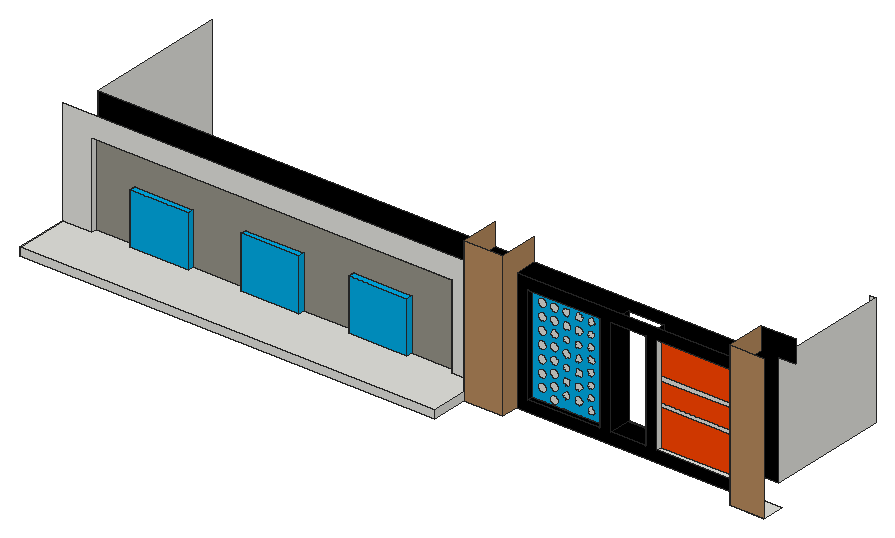
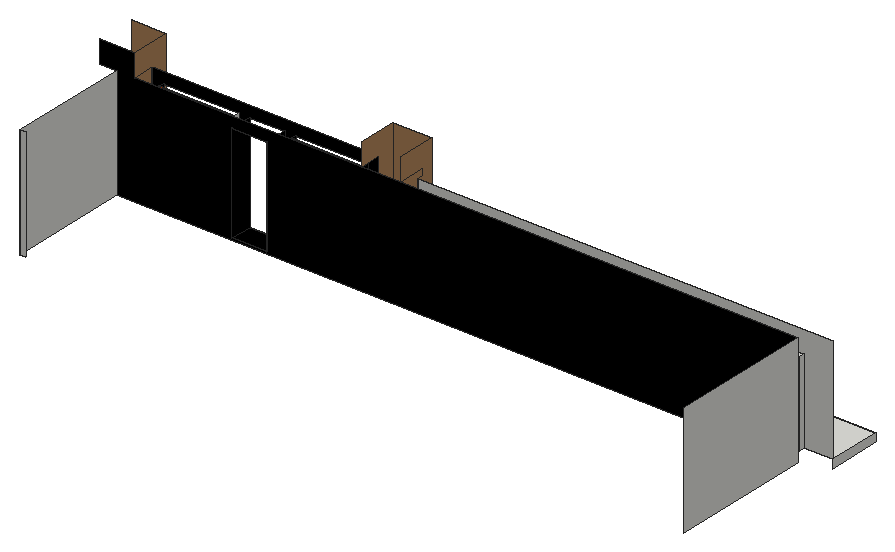
# SketchUp Ruby script. Lengths in inches.
U = 1.inch
M = Sketchup.active_model
def pt(a) = Geom::Point3d.new(a.map { |v| v * U })
def face(e, loops, mat)
  f = e.add_face(loops[0].map { |a| pt(a) })
  loops[1..].each { |l| e.add_face(l.map { |a| pt(a) }).erase! }
  f.material = f.back_material = mat if mat
  f
end
# faces: each face lists its corners as indices into pts; further lists are holes
def faces(e, pts, list, mat = nil) = list.each { |f| face(e, (f[0].is_a?(Array) ? f : [f]).map { |l| l.map { |i| pts[i] } }, mat) }
# xy, xz, yz: faces in a plane at the given z, y or x. An outline is a flat list of corners, or four numbers for a rectangle; further outlines are holes
def ring(l) = l.size == 4 ? [[l[0], l[1]], [l[2], l[1]], [l[2], l[3]], [l[0], l[3]]] : l.each_slice(2).to_a
def flat(e, list, mat, &to3) = list.each { |f| face(e, (f[0].is_a?(Array) ? f : [f]).map { |l| ring(l).map { |u, v| to3.(u, v) } }, mat) }
def xy(e, z, list, mat = nil) = flat(e, list, mat) { |x, y| [x, y, z] }
def xz(e, y, list, mat = nil) = flat(e, list, mat) { |x, z| [x, y, z] }
def yz(e, x, list, mat = nil) = flat(e, list, mat) { |y, z| [x, y, z] }
def lines(e, pts, list) = list.each { |a, b| e.add_line(pt(pts[a]), pt(pts[b])) }
# prism: a flat outline (further loops are holes) pulled along v
def prism(e, loops, v, mat = nil)
  f = face(e, loops, mat); d = Geom::Vector3d.new(v.map { |x| x * U })
  f.pushpull(f.normal.samedirection?(d) ? d.length : -d.length)
end
def box(e, o, s, mat = nil) = prism(e, [[o, [o[0] + s[0], o[1], o[2]], [o[0] + s[0], o[1] + s[1], o[2]], [o[0], o[1] + s[1], o[2]]]], [0, 0, s[2]], mat)
def at(x, y, z, deg = 0) = Geom::Transformation.translation(pt([x, y, z])) * Geom::Transformation.rotation(ORIGIN, Z_AXIS, deg.degrees)
def axes(o, x, y, z) = Geom::Transformation.new([*x, 0, *y, 0, *z, 0, *pt(o).to_a, 1])
def part(name) = M.definitions.add(name)
# library, detail: a bought-in or finely detailed component or shape, given as its bounding box
def library(name, o, s) = part(name).tap { |d| box(d.entities, o, s) }
def detail(e, o, s) = box(e.add_group.entities, o, s)
def put(e, d, t, mat = nil) = e.add_instance(d, t).tap { |i| i.material = mat if mat }
def group(e, t, mat = nil) = e.add_group.tap { |g| g.transformation = t; g.material = mat if mat }.entities
root = M.entities
M.materials.add("Niraj_Shoe_Stitching").color = [181, 137, 92]
M.materials.add("[0024_OrangeRed]").color = [255, 69, 0]
M.materials.add("[0097_DeepSkyBlue]1").color = [0, 171, 229]
M.materials.add("[0137_Black]").color = [0, 0, 0]
M.materials.add("[Formica Graystone]").color = [149, 146, 135]
xy(root,-4.9375,[[365.58,19.875,384,31.875]])
xy(root,-0.56,[[0,0,222.65,0,222.65,28.875,208.96,28.875,208.96,31.875,185.04,31.875,185.04,28.875,153.73,28.875,153.73,31.875,126.98,31.875,126.98,28.875,95.67,28.875,95.67,31.875,67.42,31.875,67.42,28.875,36.1,28.875,36.1,31.875,15.47,31.875,15.47,28.875,0,28.875]])
xy(root,1.0625,[[319.08,28.875,359.58,31.875]])
xy(root,1.0625,[[249.65,28.875,288.24,31.875],[294.24,28.875,313.08,40.875]],"[0137_Black]")
xy(root,27.07,[[36.1,28.875,67.42,31.875],[95.67,28.875,126.98,31.875],[153.73,28.875,185.04,31.875]],"[0097_DeepSkyBlue]1")
xy(root,44.57,[[15.47,28.875,208.96,31.875]])
xz(root,0,[[0,-4.9375,222.65,-0.56]])
xz(root,19.875,[[222.65,-4.9375,243.65,72],[365.58,-4.9375,384,72]],"Niraj_Shoe_Stitching")
xz(root,28.875,[[0,-0.56,15.47,-0.56,15.47,44.57,208.96,44.57,208.96,-0.56,222.65,-0.56,222.65,56.2,0,56.2]])
xz(root,28.875,[[36.1,-0.56,67.42,27.07],[95.67,-0.56,126.98,27.07],[153.73,-0.56,185.04,27.07]],"[0097_DeepSkyBlue]1")
xz(root,28.875,[[[243.65,-4.9375,365.58,60],[319.08,1.0625,359.58,54],[249.65,1.0625,288.24,54],[294.24,1.0625,313.08,54]]],"[0137_Black]")
xz(root,31.875,[[281.13,-2.54,281.62,-2.54,282.09,-2.42,282.52,-2.18,282.87,-1.83,283.11,-1.41,283.24,-0.9375,283.24,-0.45,283.12,0.03,282.875,0.45,282.53,0.8,282.11,1.05,282.05,1.0625,280.71,1.0625,280.67,1.05,280.25,0.81,279.9,0.46,279.65,0.04,279.53,-0.43,279.52,-0.92,279.65,-1.39,279.89,-1.82,280.24,-2.17,280.66,-2.41],[254.88,-1.23,255.37,-1.23,255.84,-1.11,256.27,-0.86,256.62,-0.52,256.86,-0.1,256.99,0.375,256.99,0.87,256.94,1.0625,253.33,1.0625,253.28,0.88,253.27,0.39,253.4,-0.08,253.64,-0.51,253.99,-0.85,254.41,-1.1],[274.57,-0.79,275.06,-0.79,275.53,-0.67,275.96,-0.43,276.3,-0.08,276.55,0.34,276.68,0.8125,276.68,1.0625,272.96,1.0625,272.96,0.83,273.09,0.36,273.33,-0.07,273.67,-0.42,274.1,-0.66],[268.5,-0.36,268.97,-0.23,269.39,0.01,269.74,0.36,269.99,0.78,270.07,1.0625,266.45,1.0625,266.52,0.79,266.77,0.37,267.11,0.02,267.53,-0.22,268.01,-0.35],[261.44,1.83,261.93,1.83,262.41,1.96,262.83,2.2,263.18,2.54,263.43,2.97,263.55,3.4375,263.56,3.93,263.43,4.4,263.1875,4.83,262.84,5.17,262.42,5.42,261.95,5.55,261.46,5.55,260.99,5.43,260.5625,5.18,260.21,4.84,259.97,4.42,259.84,3.94,259.84,3.46,259.96,2.98,260.2,2.56,260.55,2.21,260.97,1.96],
  [281.13,3.58,281.62,3.58,282.09,3.71,282.52,3.95,282.87,4.29,283.11,4.72,283.24,5.1875,283.24,5.68,283.12,6.15,282.875,6.58,282.53,6.92,282.11,7.17,281.64,7.3,281.15,7.3,280.67,7.18,280.25,6.93,279.9,6.59,279.65,6.17,279.53,5.69,279.52,5.21,279.65,4.73,279.89,4.31,280.24,3.96,280.66,3.71],[254.88,5.58,255.37,5.58,255.84,5.71,256.27,5.95,256.62,6.29,256.86,6.72,256.99,7.1875,256.99,7.68,256.87,8.15,256.625,8.58,256.28,8.92,255.86,9.17,255.39,9.3,254.9,9.3,254.42,9.18,254,8.93,253.65,8.59,253.4,8.17,253.28,7.69,253.27,7.21,253.4,6.73,253.64,6.31,253.99,5.96,254.41,5.71],[274.57,5.96,275.06,5.96,275.53,6.08,275.96,6.32,276.3,6.67,276.55,7.09,276.68,7.5625,276.68,8.05,276.56,8.53,276.3125,8.95,275.97,9.3,275.55,9.55,275.07,9.68,274.58,9.68,274.11,9.55,273.6875,9.31,273.34,8.96,273.09,8.54,272.96,8.07,272.96,7.58,273.09,7.11,273.33,6.68,273.67,6.33,274.1,6.09],[268.01,6.33,268.5,6.33,268.97,6.46,269.39,6.7,269.74,7.04,269.99,7.47,270.12,7.9375,270.12,8.43,269.99,8.9,269.75,9.33,269.41,9.67,268.98,9.92,268.51,10.05,268.02,10.05,267.55,9.93,267.125,9.68,266.78,9.34,266.53,8.92,266.4,8.44,266.4,7.96,266.52,7.48,266.77,7.06,267.11,6.71,267.53,6.46],[261.44,8.21,261.93,8.21,262.41,8.33,262.83,8.57,263.18,8.92,263.43,9.34,263.55,9.8125,263.56,10.3,263.43,10.78,263.1875,11.2,262.84,11.55,262.42,11.8,261.95,11.93,261.46,11.93,260.99,11.8,260.5625,11.56,260.21,11.21,259.97,10.79,259.84,10.32,259.84,9.83,259.96,9.36,260.2,8.93,260.55,8.58,260.97,8.34],
  [281.13,9.71,281.62,9.71,282.09,9.83,282.52,10.07,282.87,10.42,283.11,10.84,283.24,11.3125,283.24,11.8,283.12,12.28,282.875,12.7,282.53,13.05,282.11,13.3,281.64,13.43,281.15,13.43,280.67,13.3,280.25,13.06,279.9,12.71,279.65,12.29,279.53,11.82,279.52,11.33,279.65,10.86,279.89,10.43,280.24,10.08,280.66,9.84],[255.37,12.39,255.84,12.52,256.27,12.76,256.62,13.11,256.86,13.53,256.99,14,256.99,14.49,256.87,14.96,256.625,15.39,256.28,15.74,255.86,15.98,255.39,16.11,254.9,16.11,254.42,15.99,254,15.75,253.65,15.4,253.4,14.98,253.28,14.51,253.27,14.02,253.4,13.54,253.64,13.12,253.99,12.77,254.41,12.53,254.88,12.4],[274.57,12.71,275.06,12.71,275.53,12.83,275.96,13.07,276.3,13.42,276.55,13.84,276.68,14.3125,276.68,14.8,276.56,15.28,276.3125,15.7,275.97,16.05,275.55,16.3,275.07,16.43,274.58,16.43,274.11,16.3,273.6875,16.06,273.34,15.71,273.09,15.29,272.96,14.82,272.96,14.33,273.09,13.86,273.33,13.43,273.67,13.08,274.1,12.84],[268.01,13.02,268.5,13.02,268.97,13.14,269.39,13.39,269.74,13.73,269.99,14.15,270.12,14.625,270.12,15.12,269.99,15.59,269.75,16.01,269.41,16.36,268.98,16.61,268.51,16.74,268.02,16.74,267.55,16.61,267.125,16.37,266.78,16.03,266.53,15.6,266.4,15.13,266.4,14.64,266.52,14.17,266.77,13.74,267.11,13.4,267.53,13.15],[261.44,14.58,261.93,14.58,262.41,14.71,262.83,14.95,263.18,15.29,263.43,15.72,263.55,16.1875,263.56,16.68,263.43,17.15,263.1875,17.58,262.84,17.92,262.42,18.17,261.95,18.3,261.46,18.3,260.99,18.18,260.5625,17.93,260.21,17.59,259.97,17.17,259.84,16.69,259.84,16.21,259.96,15.73,260.2,15.31,260.55,14.96,260.97,14.71],
  [281.13,15.83,281.62,15.83,282.09,15.96,282.52,16.2,282.87,16.54,283.11,16.97,283.24,17.4375,283.24,17.93,283.12,18.4,282.875,18.83,282.53,19.17,282.11,19.42,281.64,19.55,281.15,19.55,280.67,19.43,280.25,19.18,279.9,18.84,279.65,18.42,279.53,17.94,279.52,17.46,279.65,16.98,279.89,16.56,280.24,16.21,280.66,15.96],[254.88,19.21,255.37,19.21,255.84,19.33,256.27,19.57,256.62,19.92,256.86,20.34,256.99,20.8125,256.99,21.3,256.87,21.78,256.625,22.2,256.28,22.55,255.86,22.8,255.39,22.93,254.9,22.93,254.42,22.8,254,22.56,253.65,22.21,253.4,21.79,253.28,21.32,253.27,20.83,253.4,20.36,253.64,19.93,253.99,19.58,254.41,19.34],[274.57,19.46,275.06,19.46,275.53,19.58,275.96,19.82,276.3,20.17,276.55,20.59,276.68,21.0625,276.68,21.55,276.56,22.03,276.3125,22.45,275.97,22.8,275.55,23.05,275.07,23.18,274.58,23.18,274.11,23.05,273.6875,22.81,273.34,22.46,273.09,22.04,272.96,21.57,272.96,21.08,273.09,20.61,273.33,20.18,273.67,19.83,274.1,19.59],[268.01,19.71,268.5,19.71,268.97,19.83,269.39,20.07,269.74,20.42,269.99,20.84,270.12,21.3125,270.12,21.8,269.99,22.28,269.75,22.7,269.41,23.05,268.98,23.3,268.51,23.43,268.02,23.43,267.55,23.3,267.125,23.06,266.78,22.71,266.53,22.29,266.4,21.82,266.4,21.33,266.52,20.86,266.77,20.43,267.11,20.08,267.53,19.84],[319.08,20.45,359.58,22.56],
  [261.44,20.96,261.93,20.96,262.41,21.08,262.83,21.32,263.18,21.67,263.43,22.09,263.55,22.5625,263.56,23.05,263.43,23.53,263.1875,23.95,262.84,24.3,262.42,24.55,261.95,24.68,261.46,24.68,260.99,24.55,260.5625,24.31,260.21,23.96,259.97,23.54,259.84,23.07,259.84,22.58,259.96,22.11,260.2,21.68,260.55,21.33,260.97,21.09],[281.13,21.96,281.62,21.96,282.09,22.08,282.52,22.32,282.87,22.67,283.11,23.09,283.24,23.5625,283.24,24.05,283.12,24.53,282.875,24.95,282.53,25.3,282.11,25.55,281.64,25.68,281.15,25.68,280.67,25.55,280.25,25.31,279.9,24.96,279.65,24.54,279.53,24.07,279.52,23.58,279.65,23.11,279.89,22.68,280.24,22.33,280.66,22.09],[254.88,26.02,255.37,26.02,255.84,26.14,256.27,26.39,256.62,26.73,256.86,27.15,256.99,27.625,256.99,28.12,256.87,28.59,256.625,29.01,256.28,29.36,255.86,29.61,255.39,29.74,254.9,29.74,254.42,29.61,254,29.37,253.65,29.03,253.4,28.6,253.28,28.13,253.27,27.64,253.4,27.17,253.64,26.74,253.99,26.4,254.41,26.15],[274.57,26.21,275.06,26.21,275.53,26.33,275.96,26.57,276.3,26.92,276.55,27.34,276.68,27.8125,276.68,28.3,276.56,28.78,276.3125,29.2,275.97,29.55,275.55,29.8,275.07,29.93,274.58,29.93,274.11,29.8,273.6875,29.56,273.34,29.21,273.09,28.79,272.96,28.32,272.96,27.83,273.09,27.36,273.33,26.93,273.67,26.58,274.1,26.34],[268.5,26.39,268.97,26.52,269.39,26.76,269.74,27.11,269.99,27.53,270.12,28,270.12,28.49,269.99,28.96,269.75,29.39,269.41,29.74,268.98,29.98,268.51,30.11,268.02,30.11,267.55,29.99,267.125,29.75,266.78,29.4,266.53,28.98,266.4,28.51,266.4,28.02,266.52,27.54,266.77,27.12,267.11,26.77,267.53,26.53,268.01,26.4],
  [261.44,27.33,261.93,27.33,262.41,27.46,262.83,27.7,263.18,28.04,263.43,28.47,263.55,28.9375,263.56,29.43,263.43,29.9,263.1875,30.33,262.84,30.67,262.42,30.92,261.95,31.05,261.46,31.05,260.99,30.93,260.5625,30.68,260.21,30.34,259.97,29.92,259.84,29.44,259.84,28.96,259.96,28.48,260.2,28.06,260.55,27.71,260.97,27.46],[281.13,28.08,281.62,28.08,282.09,28.21,282.52,28.45,282.87,28.79,283.11,29.22,283.24,29.6875,283.24,30.18,283.12,30.65,282.875,31.08,282.53,31.42,282.11,31.67,281.64,31.8,281.15,31.8,280.67,31.68,280.25,31.43,279.9,31.09,279.65,30.67,279.53,30.19,279.52,29.71,279.65,29.23,279.89,28.81,280.24,28.46,280.66,28.21],[254.88,32.83,255.37,32.83,255.84,32.96,256.27,33.2,256.62,33.54,256.86,33.97,256.99,34.4375,256.99,34.93,256.87,35.4,256.625,35.83,256.28,36.17,255.86,36.42,255.39,36.55,254.9,36.55,254.42,36.43,254,36.18,253.65,35.84,253.4,35.42,253.28,34.94,253.27,34.46,253.4,33.98,253.64,33.56,253.99,33.21,254.41,32.96],[274.57,32.96,275.06,32.96,275.53,33.08,275.96,33.32,276.3,33.67,276.55,34.09,276.68,34.5625,276.68,35.05,276.56,35.53,276.3125,35.95,275.97,36.3,275.55,36.55,275.07,36.68,274.58,36.68,274.11,36.55,273.6875,36.31,273.34,35.96,273.09,35.54,272.96,35.07,272.96,34.58,273.09,34.11,273.33,33.68,273.67,33.33,274.1,33.09],[268.01,33.08,268.5,33.08,268.97,33.21,269.39,33.45,269.74,33.79,269.99,34.22,270.12,34.6875,270.12,35.18,269.99,35.65,269.75,36.08,269.41,36.42,268.98,36.67,268.51,36.8,268.02,36.8,267.55,36.68,267.125,36.43,266.78,36.09,266.53,35.67,266.4,35.19,266.4,34.71,266.52,34.23,266.77,33.81,267.11,33.46,267.53,33.21],
  [319.08,33.36,359.58,35.49],[261.44,33.71,261.93,33.71,262.41,33.83,262.83,34.07,263.18,34.42,263.43,34.84,263.55,35.3125,263.56,35.8,263.43,36.28,263.1875,36.7,262.84,37.05,262.42,37.3,261.95,37.43,261.46,37.43,260.99,37.3,260.5625,37.06,260.21,36.71,259.97,36.29,259.84,35.82,259.84,35.33,259.96,34.86,260.2,34.43,260.55,34.08,260.97,33.84],[281.13,34.21,281.62,34.21,282.09,34.33,282.52,34.57,282.87,34.92,283.11,35.34,283.24,35.8125,283.24,36.3,283.12,36.78,282.875,37.2,282.53,37.55,282.11,37.8,281.64,37.93,281.15,37.93,280.67,37.8,280.25,37.56,279.9,37.21,279.65,36.79,279.53,36.32,279.52,35.83,279.65,35.36,279.89,34.93,280.24,34.58,280.66,34.34],[255.37,39.64,255.84,39.77,256.27,40.01,256.62,40.36,256.86,40.78,256.99,41.25,256.99,41.74,256.87,42.21,256.625,42.64,256.28,42.99,255.86,43.23,255.39,43.36,254.9,43.36,254.42,43.24,254,43,253.65,42.65,253.4,42.23,253.28,41.76,253.27,41.27,253.4,40.79,253.64,40.37,253.99,40.02,254.41,39.78,254.88,39.65],[274.57,39.71,275.06,39.71,275.53,39.83,275.96,40.07,276.3,40.42,276.55,40.84,276.68,41.3125,276.68,41.8,276.56,42.28,276.3125,42.7,275.97,43.05,275.55,43.3,275.07,43.43,274.58,43.43,274.11,43.3,273.6875,43.06,273.34,42.71,273.09,42.29,272.96,41.82,272.96,41.33,273.09,40.86,273.33,40.43,273.67,40.08,274.1,39.84],
  [268.01,39.77,268.5,39.77,268.97,39.89,269.39,40.14,269.74,40.48,269.99,40.9,270.12,41.375,270.12,41.87,269.99,42.34,269.75,42.76,269.41,43.11,268.98,43.36,268.51,43.49,268.02,43.49,267.55,43.36,267.125,43.12,266.78,42.78,266.53,42.35,266.4,41.88,266.4,41.39,266.52,40.92,266.77,40.49,267.11,40.15,267.53,39.9],[261.44,40.08,261.93,40.08,262.41,40.21,262.83,40.45,263.18,40.79,263.43,41.22,263.55,41.6875,263.56,42.18,263.43,42.65,263.1875,43.08,262.84,43.42,262.42,43.67,261.95,43.8,261.46,43.8,260.99,43.68,260.5625,43.43,260.21,43.09,259.97,42.67,259.84,42.19,259.84,41.71,259.96,41.23,260.2,40.81,260.55,40.46,260.97,40.21],[281.13,40.33,281.62,40.33,282.09,40.46,282.52,40.7,282.87,41.04,283.11,41.47,283.24,41.9375,283.24,42.43,283.12,42.9,282.875,43.33,282.53,43.67,282.11,43.92,281.64,44.05,281.15,44.05,280.67,43.93,280.25,43.68,279.9,43.34,279.65,42.92,279.53,42.44,279.52,41.96,279.65,41.48,279.89,41.06,280.24,40.71,280.66,40.46],[254.88,46.46,255.37,46.46,255.84,46.58,256.27,46.82,256.62,47.17,256.86,47.59,256.99,48.0625,256.99,48.55,256.87,49.03,256.625,49.45,256.28,49.8,255.86,50.05,255.39,50.18,254.9,50.18,254.42,50.05,254,49.81,253.65,49.46,253.4,49.04,253.28,48.57,253.27,48.08,253.4,47.61,253.64,47.18,253.99,46.83,254.41,46.59],[261.44,46.46,261.93,46.46,262.41,46.58,262.83,46.82,263.18,47.17,263.43,47.59,263.55,48.0625,263.56,48.55,263.43,49.03,263.1875,49.45,262.84,49.8,262.42,50.05,261.95,50.18,261.46,50.18,260.99,50.05,260.5625,49.81,260.21,49.46,259.97,49.04,259.84,48.57,259.84,48.08,259.96,47.61,260.2,47.18,260.55,46.83,260.97,46.59],
  [268.01,46.46,268.5,46.46,268.97,46.58,269.39,46.82,269.74,47.17,269.99,47.59,270.12,48.0625,270.12,48.55,269.99,49.03,269.75,49.45,269.41,49.8,268.98,50.05,268.51,50.18,268.02,50.18,267.55,50.05,267.125,49.81,266.78,49.46,266.53,49.04,266.4,48.57,266.4,48.08,266.52,47.61,266.77,47.18,267.11,46.83,267.53,46.59],[274.57,46.46,275.06,46.46,275.53,46.58,275.96,46.82,276.3,47.17,276.55,47.59,276.68,48.0625,276.68,48.55,276.56,49.03,276.3125,49.45,275.97,49.8,275.55,50.05,275.07,50.18,274.58,50.18,274.11,50.05,273.6875,49.81,273.34,49.46,273.09,49.04,272.96,48.57,272.96,48.08,273.09,47.61,273.33,47.18,273.67,46.83,274.1,46.59],[281.13,46.46,281.62,46.46,282.09,46.58,282.52,46.82,282.87,47.17,283.11,47.59,283.24,48.0625,283.24,48.55,283.12,49.03,282.875,49.45,282.53,49.8,282.11,50.05,281.64,50.18,281.15,50.18,280.67,50.05,280.25,49.81,279.9,49.46,279.65,49.04,279.53,48.57,279.52,48.08,279.65,47.61,279.89,47.18,280.24,46.83,280.66,46.59],[288.24,46.47,288.66,46.58,289.08,46.82,289.43,47.17,289.68,47.59,289.8,48.0625,289.81,48.55,289.68,49.03,289.4375,49.45,289.09,49.8,288.67,50.05,288.24,50.16]])
xz(root,31.875,[[319.08,1.0625,359.58,20.45],[319.08,22.56,359.58,33.36],[319.08,35.49,359.58,54]],"[0024_OrangeRed]")
xz(root,31.875,[[[249.65,1.0625,288.24,54],[261.44,46.46,260.97,46.59,260.55,46.83,260.2,47.18,259.96,47.61,259.84,48.08,259.84,48.57,259.97,49.04,260.21,49.46,260.5625,49.81,260.99,50.05,261.46,50.18,261.95,50.18,262.42,50.05,262.84,49.8,263.1875,49.45,263.43,49.03,263.56,48.55,263.55,48.0625,263.43,47.59,263.18,47.17,262.83,46.82,262.41,46.58,261.93,46.46],[268.01,46.46,267.53,46.59,267.11,46.83,266.77,47.18,266.52,47.61,266.4,48.08,266.4,48.57,266.53,49.04,266.78,49.46,267.125,49.81,267.55,50.05,268.02,50.18,268.51,50.18,268.98,50.05,269.41,49.8,269.75,49.45,269.99,49.03,270.12,48.55,270.12,48.0625,269.99,47.59,269.74,47.17,269.39,46.82,268.97,46.58,268.5,46.46],[274.57,46.46,274.1,46.59,273.67,46.83,273.33,47.18,273.09,47.61,272.96,48.08,272.96,48.57,273.09,49.04,273.34,49.46,273.6875,49.81,274.11,50.05,274.58,50.18,275.07,50.18,275.55,50.05,275.97,49.8,276.3125,49.45,276.56,49.03,276.68,48.55,276.68,48.0625,276.55,47.59,276.3,47.17,275.96,46.82,275.53,46.58,275.06,46.46],[281.13,46.46,280.66,46.59,280.24,46.83,279.89,47.18,279.65,47.61,279.52,48.08,279.53,48.57,279.65,49.04,279.9,49.46,280.25,49.81,280.67,50.05,281.15,50.18,281.64,50.18,282.11,50.05,282.53,49.8,282.875,49.45,283.12,49.03,283.24,48.55,283.24,48.0625,283.11,47.59,282.87,47.17,282.52,46.82,282.09,46.58,281.62,46.46],[281.13,40.33,280.66,40.46,280.24,40.71,279.89,41.06,279.65,41.48,279.52,41.96,279.53,42.44,279.65,42.92,279.9,43.34,280.25,43.68,280.67,43.93,281.15,44.05,281.64,44.05,282.11,43.92,282.53,43.67,282.875,43.33,283.12,42.9,283.24,42.43,283.24,41.9375,283.11,41.47,282.87,41.04,282.52,40.7,282.09,40.46,281.62,40.33],[281.13,34.21,280.66,34.34,280.24,34.58,279.89,34.93,279.65,35.36,279.52,35.83,279.53,36.32,279.65,36.79,279.9,37.21,280.25,37.56,280.67,37.8,281.15,37.93,281.64,37.93,282.11,37.8,282.53,37.55,282.875,37.2,283.12,36.78,283.24,36.3,283.24,35.8125,283.11,35.34,282.87,34.92,282.52,34.57,282.09,34.33,281.62,34.21],[281.13,28.08,280.66,28.21,280.24,28.46,279.89,28.81,279.65,29.23,279.52,29.71,279.53,30.19,279.65,30.67,279.9,31.09,280.25,31.43,280.67,31.68,281.15,31.8,281.64,31.8,282.11,31.67,282.53,31.42,282.875,31.08,283.12,30.65,283.24,30.18,283.24,29.6875,283.11,29.22,282.87,28.79,282.52,28.45,282.09,28.21,281.62,28.08],[281.13,21.96,280.66,22.09,280.24,22.33,279.89,22.68,279.65,23.11,279.52,23.58,279.53,24.07,279.65,24.54,279.9,24.96,280.25,25.31,280.67,25.55,281.15,25.68,281.64,25.68,282.11,25.55,282.53,25.3,282.875,24.95,283.12,24.53,283.24,24.05,283.24,23.5625,283.11,23.09,282.87,22.67,282.52,22.32,282.09,22.08,281.62,21.96],[281.13,15.83,280.66,15.96,280.24,16.21,279.89,16.56,279.65,16.98,279.52,17.46,279.53,17.94,279.65,18.42,279.9,18.84,280.25,19.18,280.67,19.43,281.15,19.55,281.64,19.55,282.11,19.42,282.53,19.17,282.875,18.83,283.12,18.4,283.24,17.93,283.24,17.4375,283.11,16.97,282.87,16.54,282.52,16.2,282.09,15.96,281.62,15.83],[281.13,9.71,280.66,9.84,280.24,10.08,279.89,10.43,279.65,10.86,279.52,11.33,279.53,11.82,279.65,12.29,279.9,12.71,280.25,13.06,280.67,13.3,281.15,13.43,281.64,13.43,282.11,13.3,282.53,13.05,282.875,12.7,283.12,12.28,283.24,11.8,283.24,11.3125,283.11,10.84,282.87,10.42,282.52,10.07,282.09,9.83,281.62,9.71],[281.13,3.58,280.66,3.71,280.24,3.96,279.89,4.31,279.65,4.73,279.52,5.21,279.53,5.69,279.65,6.17,279.9,6.59,280.25,6.93,280.67,7.18,281.15,7.3,281.64,7.3,282.11,7.17,282.53,6.92,282.875,6.58,283.12,6.15,283.24,5.68,283.24,5.1875,283.11,4.72,282.87,4.29,282.52,3.95,282.09,3.71,281.62,3.58],[274.57,39.71,274.1,39.84,273.67,40.08,273.33,40.43,273.09,40.86,272.96,41.33,272.96,41.82,273.09,42.29,273.34,42.71,273.6875,43.06,274.11,43.3,274.58,43.43,275.07,43.43,275.55,43.3,275.97,43.05,276.3125,42.7,276.56,42.28,276.68,41.8,276.68,41.3125,276.55,40.84,276.3,40.42,275.96,40.07,275.53,39.83,275.06,39.71],[274.57,32.96,274.1,33.09,273.67,33.33,273.33,33.68,273.09,34.11,272.96,34.58,272.96,35.07,273.09,35.54,273.34,35.96,273.6875,36.31,274.11,36.55,274.58,36.68,275.07,36.68,275.55,36.55,275.97,36.3,276.3125,35.95,276.56,35.53,276.68,35.05,276.68,34.5625,276.55,34.09,276.3,33.67,275.96,33.32,275.53,33.08,275.06,32.96],[274.57,26.21,274.1,26.34,273.67,26.58,273.33,26.93,273.09,27.36,272.96,27.83,272.96,28.32,273.09,28.79,273.34,29.21,273.6875,29.56,274.11,29.8,274.58,29.93,275.07,29.93,275.55,29.8,275.97,29.55,276.3125,29.2,276.56,28.78,276.68,28.3,276.68,27.8125,276.55,27.34,276.3,26.92,275.96,26.57,275.53,26.33,275.06,26.21],[274.57,19.46,274.1,19.59,273.67,19.83,273.33,20.18,273.09,20.61,272.96,21.08,272.96,21.57,273.09,22.04,273.34,22.46,273.6875,22.81,274.11,23.05,274.58,23.18,275.07,23.18,275.55,23.05,275.97,22.8,276.3125,22.45,276.56,22.03,276.68,21.55,276.68,21.0625,276.55,20.59,276.3,20.17,275.96,19.82,275.53,19.58,275.06,19.46],[274.57,12.71,274.1,12.84,273.67,13.08,273.33,13.43,273.09,13.86,272.96,14.33,272.96,14.82,273.09,15.29,273.34,15.71,273.6875,16.06,274.11,16.3,274.58,16.43,275.07,16.43,275.55,16.3,275.97,16.05,276.3125,15.7,276.56,15.28,276.68,14.8,276.68,14.3125,276.55,13.84,276.3,13.42,275.96,13.07,275.53,12.83,275.06,12.71],[274.57,5.96,274.1,6.09,273.67,6.33,273.33,6.68,273.09,7.11,272.96,7.58,272.96,8.07,273.09,8.54,273.34,8.96,273.6875,9.31,274.11,9.55,274.58,9.68,275.07,9.68,275.55,9.55,275.97,9.3,276.3125,8.95,276.56,8.53,276.68,8.05,276.68,7.5625,276.55,7.09,276.3,6.67,275.96,6.32,275.53,6.08,275.06,5.96],[268.01,39.77,267.53,39.9,267.11,40.15,266.77,40.49,266.52,40.92,266.4,41.39,266.4,41.88,266.53,42.35,266.78,42.78,267.125,43.12,267.55,43.36,268.02,43.49,268.51,43.49,268.98,43.36,269.41,43.11,269.75,42.76,269.99,42.34,270.12,41.87,270.12,41.375,269.99,40.9,269.74,40.48,269.39,40.14,268.97,39.89,268.5,39.77],[268.01,33.08,267.53,33.21,267.11,33.46,266.77,33.81,266.52,34.23,266.4,34.71,266.4,35.19,266.53,35.67,266.78,36.09,267.125,36.43,267.55,36.68,268.02,36.8,268.51,36.8,268.98,36.67,269.41,36.42,269.75,36.08,269.99,35.65,270.12,35.18,270.12,34.6875,269.99,34.22,269.74,33.79,269.39,33.45,268.97,33.21,268.5,33.08],[268.5,26.39,268.01,26.4,267.53,26.53,267.11,26.77,266.77,27.12,266.52,27.54,266.4,28.02,266.4,28.51,266.53,28.98,266.78,29.4,267.125,29.75,267.55,29.99,268.02,30.11,268.51,30.11,268.98,29.98,269.41,29.74,269.75,29.39,269.99,28.96,270.12,28.49,270.12,28,269.99,27.53,269.74,27.11,269.39,26.76,268.97,26.52],[268.01,19.71,267.53,19.84,267.11,20.08,266.77,20.43,266.52,20.86,266.4,21.33,266.4,21.82,266.53,22.29,266.78,22.71,267.125,23.06,267.55,23.3,268.02,23.43,268.51,23.43,268.98,23.3,269.41,23.05,269.75,22.7,269.99,22.28,270.12,21.8,270.12,21.3125,269.99,20.84,269.74,20.42,269.39,20.07,268.97,19.83,268.5,19.71],[268.01,13.02,267.53,13.15,267.11,13.4,266.77,13.74,266.52,14.17,266.4,14.64,266.4,15.13,266.53,15.6,266.78,16.03,267.125,16.37,267.55,16.61,268.02,16.74,268.51,16.74,268.98,16.61,269.41,16.36,269.75,16.01,269.99,15.59,270.12,15.12,270.12,14.625,269.99,14.15,269.74,13.73,269.39,13.39,268.97,13.14,268.5,13.02],[268.01,6.33,267.53,6.46,267.11,6.71,266.77,7.06,266.52,7.48,266.4,7.96,266.4,8.44,266.53,8.92,266.78,9.34,267.125,9.68,267.55,9.93,268.02,10.05,268.51,10.05,268.98,9.92,269.41,9.67,269.75,9.33,269.99,8.9,270.12,8.43,270.12,7.9375,269.99,7.47,269.74,7.04,269.39,6.7,268.97,6.46,268.5,6.33],[255.37,39.64,254.88,39.65,254.41,39.78,253.99,40.02,253.64,40.37,253.4,40.79,253.27,41.27,253.28,41.76,253.4,42.23,253.65,42.65,254,43,254.42,43.24,254.9,43.36,255.39,43.36,255.86,43.23,256.28,42.99,256.625,42.64,256.87,42.21,256.99,41.74,256.99,41.25,256.86,40.78,256.62,40.36,256.27,40.01,255.84,39.77],[254.88,32.83,254.41,32.96,253.99,33.21,253.64,33.56,253.4,33.98,253.27,34.46,253.28,34.94,253.4,35.42,253.65,35.84,254,36.18,254.42,36.43,254.9,36.55,255.39,36.55,255.86,36.42,256.28,36.17,256.625,35.83,256.87,35.4,256.99,34.93,256.99,34.4375,256.86,33.97,256.62,33.54,256.27,33.2,255.84,32.96,255.37,32.83],[254.88,26.02,254.41,26.15,253.99,26.4,253.64,26.74,253.4,27.17,253.27,27.64,253.28,28.13,253.4,28.6,253.65,29.03,254,29.37,254.42,29.61,254.9,29.74,255.39,29.74,255.86,29.61,256.28,29.36,256.625,29.01,256.87,28.59,256.99,28.12,256.99,27.625,256.86,27.15,256.62,26.73,256.27,26.39,255.84,26.14,255.37,26.02],[254.88,19.21,254.41,19.34,253.99,19.58,253.64,19.93,253.4,20.36,253.27,20.83,253.28,21.32,253.4,21.79,253.65,22.21,254,22.56,254.42,22.8,254.9,22.93,255.39,22.93,255.86,22.8,256.28,22.55,256.625,22.2,256.87,21.78,256.99,21.3,256.99,20.8125,256.86,20.34,256.62,19.92,256.27,19.57,255.84,19.33,255.37,19.21],[255.37,12.39,254.88,12.4,254.41,12.53,253.99,12.77,253.64,13.12,253.4,13.54,253.27,14.02,253.28,14.51,253.4,14.98,253.65,15.4,254,15.75,254.42,15.99,254.9,16.11,255.39,16.11,255.86,15.98,256.28,15.74,256.625,15.39,256.87,14.96,256.99,14.49,256.99,14,256.86,13.53,256.62,13.11,256.27,12.76,255.84,12.52],[254.88,5.58,254.41,5.71,253.99,5.96,253.64,6.31,253.4,6.73,253.27,7.21,253.28,7.69,253.4,8.17,253.65,8.59,254,8.93,254.42,9.18,254.9,9.3,255.39,9.3,255.86,9.17,256.28,8.92,256.625,8.58,256.87,8.15,256.99,7.68,256.99,7.1875,256.86,6.72,256.62,6.29,256.27,5.95,255.84,5.71,255.37,5.58],[261.44,40.08,260.97,40.21,260.55,40.46,260.2,40.81,259.96,41.23,259.84,41.71,259.84,42.19,259.97,42.67,260.21,43.09,260.5625,43.43,260.99,43.68,261.46,43.8,261.95,43.8,262.42,43.67,262.84,43.42,263.1875,43.08,263.43,42.65,263.56,42.18,263.55,41.6875,263.43,41.22,263.18,40.79,262.83,40.45,262.41,40.21,261.93,40.08],[261.44,33.71,260.97,33.84,260.55,34.08,260.2,34.43,259.96,34.86,259.84,35.33,259.84,35.82,259.97,36.29,260.21,36.71,260.5625,37.06,260.99,37.3,261.46,37.43,261.95,37.43,262.42,37.3,262.84,37.05,263.1875,36.7,263.43,36.28,263.56,35.8,263.55,35.3125,263.43,34.84,263.18,34.42,262.83,34.07,262.41,33.83,261.93,33.71],[261.44,27.33,260.97,27.46,260.55,27.71,260.2,28.06,259.96,28.48,259.84,28.96,259.84,29.44,259.97,29.92,260.21,30.34,260.5625,30.68,260.99,30.93,261.46,31.05,261.95,31.05,262.42,30.92,262.84,30.67,263.1875,30.33,263.43,29.9,263.56,29.43,263.55,28.9375,263.43,28.47,263.18,28.04,262.83,27.7,262.41,27.46,261.93,27.33],[261.44,20.96,260.97,21.09,260.55,21.33,260.2,21.68,259.96,22.11,259.84,22.58,259.84,23.07,259.97,23.54,260.21,23.96,260.5625,24.31,260.99,24.55,261.46,24.68,261.95,24.68,262.42,24.55,262.84,24.3,263.1875,23.95,263.43,23.53,263.56,23.05,263.55,22.5625,263.43,22.09,263.18,21.67,262.83,21.32,262.41,21.08,261.93,20.96],[261.44,14.58,260.97,14.71,260.55,14.96,260.2,15.31,259.96,15.73,259.84,16.21,259.84,16.69,259.97,17.17,260.21,17.59,260.5625,17.93,260.99,18.18,261.46,18.3,261.95,18.3,262.42,18.17,262.84,17.92,263.1875,17.58,263.43,17.15,263.56,16.68,263.55,16.1875,263.43,15.72,263.18,15.29,262.83,14.95,262.41,14.71,261.93,14.58],[261.44,8.21,260.97,8.34,260.55,8.58,260.2,8.93,259.96,9.36,259.84,9.83,259.84,10.32,259.97,10.79,260.21,11.21,260.5625,11.56,260.99,11.8,261.46,11.93,261.95,11.93,262.42,11.8,262.84,11.55,263.1875,11.2,263.43,10.78,263.56,10.3,263.55,9.8125,263.43,9.34,263.18,8.92,262.83,8.57,262.41,8.33,261.93,8.21],[261.44,1.83,260.97,1.96,260.55,2.21,260.2,2.56,259.96,2.98,259.84,3.46,259.84,3.94,259.97,4.42,260.21,4.84,260.5625,5.18,260.99,5.43,261.46,5.55,261.95,5.55,262.42,5.42,262.84,5.17,263.1875,4.83,263.43,4.4,263.56,3.93,263.55,3.4375,263.43,2.97,263.18,2.54,262.83,2.2,262.41,1.96,261.93,1.83],[254.88,46.46,254.41,46.59,253.99,46.83,253.64,47.18,253.4,47.61,253.27,48.08,253.28,48.57,253.4,49.04,253.65,49.46,254,49.81,254.42,50.05,254.9,50.18,255.39,50.18,255.86,50.05,256.28,49.8,256.625,49.45,256.87,49.03,256.99,48.55,256.99,48.0625,256.86,47.59,256.62,47.17,256.27,46.82,255.84,46.58,255.37,46.46]]],"[0097_DeepSkyBlue]1")
xz(root,31.875,[[15.47,-0.56,36.1,-0.56,36.1,27.07,67.42,27.07,67.42,-0.56,95.67,-0.56,95.67,27.07,126.98,27.07,126.98,-0.56,153.73,-0.56,153.73,27.07,185.04,27.07,185.04,-0.56,208.96,-0.56,208.96,44.57,15.47,44.57]],"[Formica Graystone]")
xz(root,40.875,[[[9,0,9,60,365.58,60,365.58,72,384,72,384,60,375,60,375,0],[294.24,1.0625,313.08,54]]],"[0137_Black]")
xz(root,106,[[372,0,375,60]])
yz(root,0,[[0,-4.9375,28.875,-0.56]])
yz(root,9,[[40.875,0,117.875,60]])
yz(root,15.47,[[28.875,-0.56,31.875,44.57]])
yz(root,36.1,[[28.875,-0.56,31.875,27.07]],"[0097_DeepSkyBlue]1")
yz(root,67.42,[[28.875,-0.56,31.875,27.07]],"[0097_DeepSkyBlue]1")
yz(root,95.67,[[28.875,-0.56,31.875,27.07]],"[0097_DeepSkyBlue]1")
yz(root,126.98,[[28.875,-0.56,31.875,27.07]],"[0097_DeepSkyBlue]1")
yz(root,153.73,[[28.875,-0.56,31.875,27.07]],"[0097_DeepSkyBlue]1")
yz(root,185.04,[[28.875,-0.56,31.875,27.07]],"[0097_DeepSkyBlue]1")
yz(root,208.96,[[28.875,-0.56,31.875,44.57]])
yz(root,222.65,[[0,-4.9375,19.875,-0.56]])
yz(root,222.65,[[19.875,-0.56,19.875,72,40.875,72,40.875,60,25.875,60,25.875,56.2,28.875,56.2,28.875,-0.56]],"Niraj_Shoe_Stitching")
yz(root,243.65,[[19.875,-4.9375,28.875,-4.9375,28.875,60,40.875,60,40.875,72,19.875,72]],"Niraj_Shoe_Stitching")
yz(root,249.65,[[28.875,1.0625,31.875,54]],"[0137_Black]")
yz(root,288.24,[[28.875,1.0625,31.875,54]],"[0137_Black]")
yz(root,294.24,[[28.875,1.0625,40.875,54]],"[0137_Black]")
yz(root,313.08,[[28.875,1.0625,40.875,54]],"[0137_Black]")
yz(root,319.08,[[28.875,1.0625,31.875,54]])
yz(root,359.58,[[28.875,1.0625,31.875,54]],"[0137_Black]")
yz(root,365.58,[[19.875,-4.9375,19.875,72,40.875,72,40.875,60,28.875,60,28.875,-4.9375]],"Niraj_Shoe_Stitching")
yz(root,375,[[40.875,0,106,60]])
p = [[208.96,31.875,-4.9375],[208.96,31.875,-0.56],[15.47,31.875,-0.56],[15.47,31.875,-4.9375],[15.47,28.875,-0.56],[15.47,28.875,-4.9375],
  [222.65,28.875,-0.56],[222.65,28.875,-4.9375],[259.96,31.875,-3.39],[259.84,31.875,-2.92],[262.84,31.875,-1.2],[263.1875,31.875,-1.55],
  [263.43,31.875,-1.97],[263.56,31.875,-2.45],[263.55,31.875,-2.9375],[263.43,31.875,-3.41],[263.18,31.875,-3.83],[262.83,31.875,-4.18],
  [262.41,31.875,-4.42],[261.93,31.875,-4.54],[261.44,31.875,-4.54],[260.97,31.875,-4.41],[260.55,31.875,-4.17],[260.2,31.875,-3.82],
  [259.84,31.875,-2.43],[259.97,31.875,-1.96],[260.21,31.875,-1.54],[260.5625,31.875,-1.19],[260.99,31.875,-0.95],[261.46,31.875,-0.82],
  [261.95,31.875,-0.82],[262.42,31.875,-0.95]]
lines(root,p,[[0,1],[2,3],[4,5],[6,7],[8,9],[10,11],[11,12],[12,13],[13,14],[14,15],[15,16],[16,17],
  [17,18],[18,19],[19,20],[20,21],[21,22],[22,23],[23,8],[9,24],[24,25],[25,26],[26,27],[27,28],
  [28,29],[29,30],[30,31],[31,10]])
